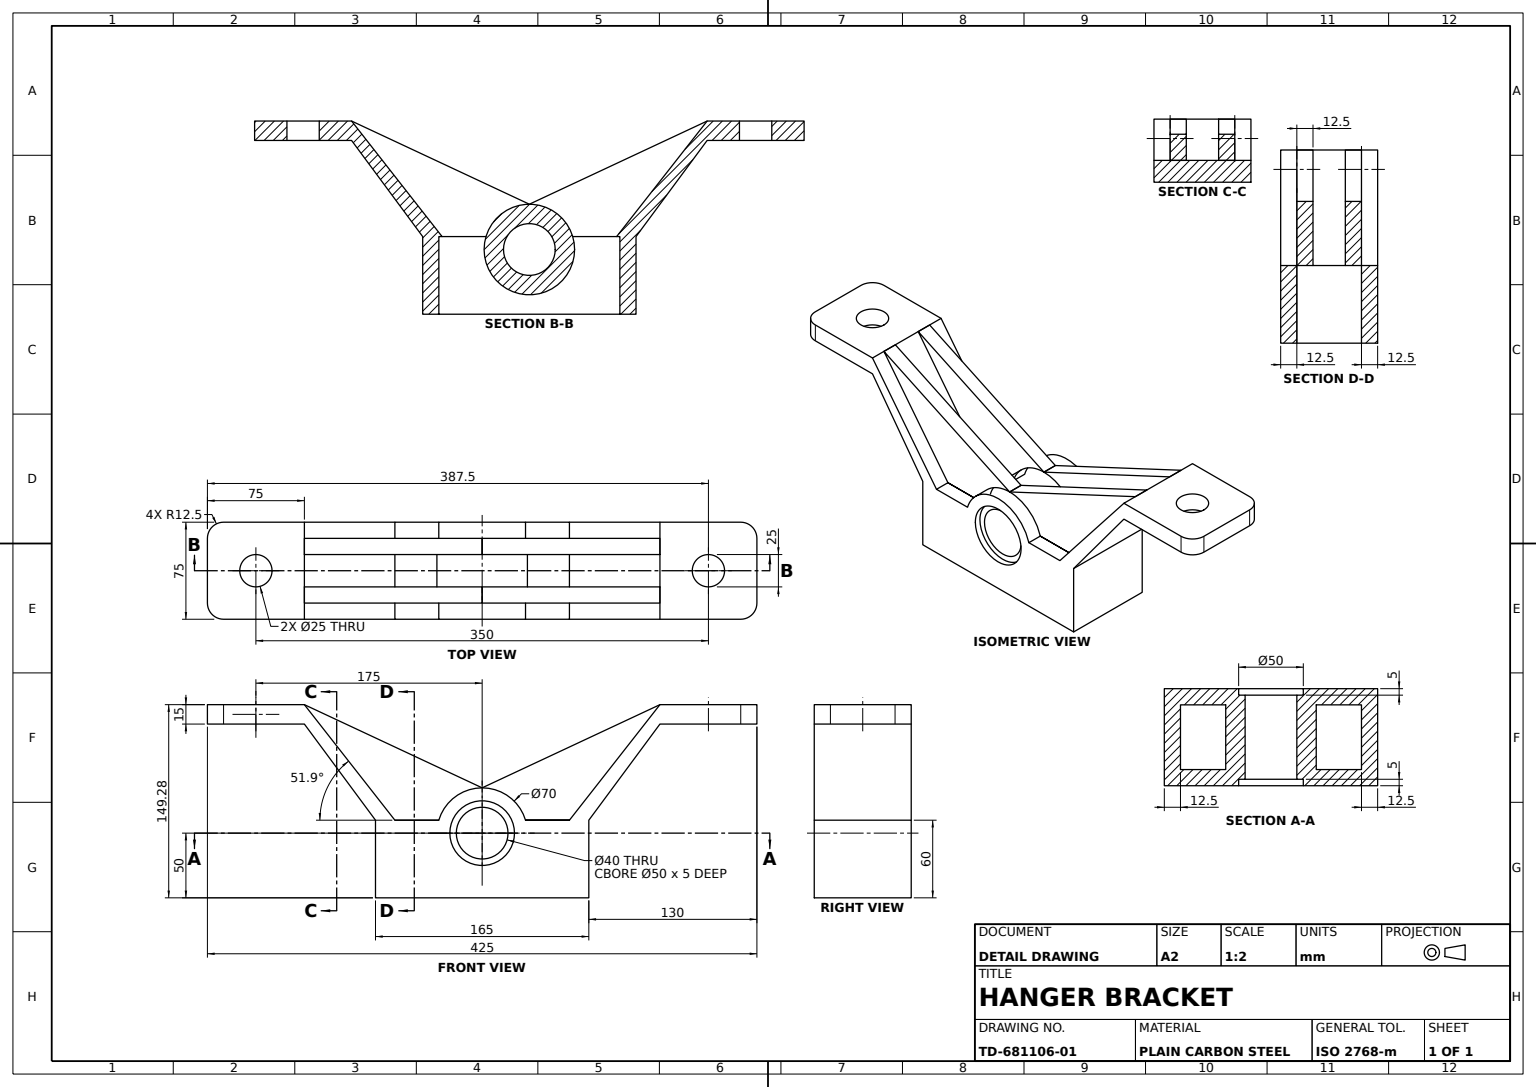
solid
v1 (-137.5,149.280992,12.5)
v2 (-67.5,60,12.5)
e1 v1 v2 LINE
v3 (0,85,12.5)
e2 v3 v1 LINE
v4 (-33.54102,60,12.5)
e3 v4 v3 CIRCLE(AX(P(0,50,12.5),D(0,0,-1),D(-1,0,0)),35)
e4 v2 v4 LINE
face PLANE(AX(P(0,50,12.5),D(0,0,-1),D(-1,0,0))) [-e1 -e2 -e3 -e4]
v5 (-137.5,149.280992,25)
v6 (-67.5,60,25)
e5 v5 v6 LINE
e6 v1 v5 LINE
e7 v2 v6 LINE
face PLANE(AX(P(-137.5,149.280992,12.5),D(-0.786957449,-0.617007272,0),D(0.617007272,-0.786957449,0))) [-e5 -e6 e1 e7]
v7 (0,85,25)
e8 v3 v7 LINE
v8 (-33.54102,60,25)
e9 v8 v7 CIRCLE(AX(P(0,50,25),D(0,0,-1),D(-1,0,0)),35)
e10 v4 v8 LINE
face CYL(AX(P(0,50,12.5),D(0,0,1),D(1,0,0)),35) rev [e3 e8 -e9 -e10]
e11 v7 v5 LINE
e12 v6 v8 LINE
face PLANE(AX(P(0,50,25),D(0,0,-1),D(-1,0,0))) rev [e11 e5 e12 e9]
face PLANE(AX(P(-137.5,149.280992,12.5),D(0.423503881,0.905894289,0),D(-0.905894289,0.423503881,0))) [-e8 e2 e6 -e11]
face PLANE(AX(P(-67.5,60,12.5),D(0,-1,0),D(0,0,-1))) [e4 e10 -e12 -e7]
solid
v9 (137.5,149.280992,-12.5)
v10 (137.5,149.280992,-25)
e13 v9 v10 LINE
v11 (67.5,60,-12.5)
e14 v9 v11 LINE
v12 (67.5,60,-25)
e15 v11 v12 LINE
e16 v10 v12 LINE
face PLANE(AX(P(137.5,149.280992,-12.5),D(0.786957449,-0.617007272,0),D(-0.617007272,-0.786957449,0))) [-e13 e14 e15 -e16]
v13 (0,85,-12.5)
e17 v13 v9 LINE
v14 (33.54102,60,-12.5)
e18 v14 v13 CIRCLE(AX(P(0,50,-12.5),D(0,0,1),D(1,0,0)),35)
e19 v11 v14 LINE
face PLANE(AX(P(0,50,-12.5),D(0,0,1),D(1,0,0))) [-e14 -e17 -e18 -e19]
v15 (0,85,-25)
e20 v15 v10 LINE
e21 v13 v15 LINE
face PLANE(AX(P(137.5,149.280992,-12.5),D(-0.423503881,0.905894289,0),D(0.905894289,0.423503881,0))) [e17 e13 -e20 -e21]
v16 (33.54102,60,-25)
e22 v16 v15 CIRCLE(AX(P(0,50,-25),D(0,0,1),D(1,0,0)),35)
e23 v14 v16 LINE
face CYL(AX(P(0,50,-12.5),D(0,0,-1),D(-1,0,0)),35) rev [e21 -e22 -e23 e18]
e24 v12 v16 LINE
face PLANE(AX(P(67.5,60,-12.5),D(0,-1,0),D(0,0,1))) [-e24 -e15 e19 e23]
face PLANE(AX(P(0,50,-25),D(0,0,1),D(1,0,0))) rev [e20 e16 e24 e22]
solid
v17 (-200,149.280992,37.5)
v18 (-200,134.280992,37.5)
e25 v17 v18 LINE
v19 (-212.5,149.280992,25)
e26 v19 v17 CIRCLE(AX(P(-200,149.280992,25),D(0,1,0),D(-1,0,0)),12.5)
v20 (-212.5,134.280992,25)
e27 v20 v19 LINE
e28 v18 v20 CIRCLE(AX(P(-200,134.280992,25),D(0,-1,0),D(0,0,-1)),12.5)
face CYL(AX(P(-200,60,25),D(0,1,0),D(0,0,1)),12.5) [-e25 -e26 -e27 -e28]
v21 (-187.5,134.280992,0)
v22 (-162.5,134.280992,0)
e29 v21 v22 CIRCLE(AX(P(-175,134.280992,0),D(0,-1,0),D(0,0,-1)),12.5)
e30 v22 v21 CIRCLE(AX(P(-175,134.280992,0),D(0,-1,0),D(0,0,-1)),12.5)
v23 (-212.5,134.280992,-25)
e31 v23 v20 LINE
v24 (-200,134.280992,-37.5)
e32 v23 v24 CIRCLE(AX(P(-200,134.280992,-25),D(0,-1,0),D(0,0,-1)),12.5)
v25 (-137.5,134.280992,-37.5)
e33 v24 v25 LINE
v26 (-137.5,134.280992,37.5)
e34 v25 v26 LINE
e35 v18 v26 LINE
face PLANE(AX(P(-212.5,134.280992,-37.5),D(0,-1,0),D(0,0,-1))) [-e29 -e30] [e28 -e31 e32 e33 e34 -e35]
v27 (-67.5,60,37.5)
v28 (-33.54102,60,37.5)
e36 v27 v28 LINE
v29 (-33.54102,60,25)
e37 v29 v28 LINE
v30 (-67.5,60,25)
e38 v30 v29 LINE
e39 v30 v27 LINE
face PLANE(AX(P(0,60,0),D(0,1,0),D(0,0,1))) [e36 -e37 -e38 e39]
v31 (-187.5,149.280992,0)
v32 (-162.5,149.280992,0)
e40 v31 v32 CIRCLE(AX(P(-175,149.280992,0),D(0,1,0),D(-1,0,0)),12.5)
e41 v32 v31 CIRCLE(AX(P(-175,149.280992,0),D(0,1,0),D(-1,0,0)),12.5)
v33 (-212.5,149.280992,-25)
e42 v33 v19 LINE
v34 (-137.5,149.280992,37.5)
e43 v34 v17 LINE
v35 (-137.5,149.280992,-37.5)
e44 v35 v34 LINE
v36 (-200,149.280992,-37.5)
e45 v35 v36 LINE
e46 v36 v33 CIRCLE(AX(P(-200,149.280992,-25),D(0,1,0),D(-1,0,0)),12.5)
face PLANE(AX(P(-137.5,149.280992,-37.5),D(0,1,0),D(-1,0,0))) [-e40 -e41] [e42 e26 -e43 -e44 e45 e46]
v37 (25,50,32.5)
v38 (-25,50,32.5)
e47 v37 v38 CIRCLE(AX(P(0,50,32.5),D(0,0,1),D(1,0,0)),25)
e48 v38 v37 CIRCLE(AX(P(0,50,32.5),D(0,0,1),D(1,0,0)),25)
v39 (-20,50,32.5)
v40 (20,50,32.5)
e49 v39 v40 CIRCLE(AX(P(0,50,32.5),D(0,0,1),D(1,0,0)),20)
e50 v40 v39 CIRCLE(AX(P(0,50,32.5),D(0,0,1),D(1,0,0)),20)
face PLANE(AX(P(0,50,32.5),D(0,0,1),D(1,0,0))) [e47 e48] [-e49 -e50]
v41 (-70,60,-25)
v42 (-70,60,25)
e51 v41 v42 LINE
v43 (-67.5,60,-25)
e52 v43 v41 LINE
e53 v43 v30 LINE
e54 v42 v30 LINE
face PLANE(AX(P(-82.5,60,-37.5),D(0,-1,0),D(0,0,-1))) [-e51 -e52 e53 -e54]
e55 v33 v23 LINE
face PLANE(AX(P(-212.5,149.280992,-37.5),D(-1,0,0),D(0,0,1))) [e31 e27 -e42 e55]
v44 (-20,50,-32.5)
e56 v44 v39 LINE
v45 (20,50,-32.5)
e57 v45 v40 LINE
e58 v44 v45 CIRCLE(AX(P(0,50,-32.5),D(0,0,1),D(-1,0,0)),20)
face CYL(AX(P(0,50,-76.5),D(0,0,1),D(1,0,0)),20) rev [e56 e49 -e57 -e58]
e59 v45 v44 CIRCLE(AX(P(0,50,-32.5),D(0,0,1),D(-1,0,0)),20)
face CYL(AX(P(0,50,-76.5),D(0,0,1),D(1,0,0)),20) rev [-e59 e57 e50 -e56]
v46 (-25,50,37.5)
e60 v38 v46 LINE
v47 (25,50,37.5)
e61 v37 v47 LINE
e62 v47 v46 CIRCLE(AX(P(0,50,37.5),D(0,0,1),D(1,0,0)),25)
face CYL(AX(P(0,50,32.5),D(0,0,1),D(1,0,0)),25) rev [-e60 -e47 e61 e62]
v48 (-70,0,25)
v49 (70,0,25)
e63 v48 v49 LINE
v50 (70,0,-25)
e64 v49 v50 LINE
v51 (-70,0,-25)
e65 v50 v51 LINE
e66 v51 v48 LINE
v52 (82.5,0,37.5)
v53 (82.5,0,-37.5)
e67 v52 v53 LINE
v54 (-82.5,0,37.5)
e68 v54 v52 LINE
v55 (-82.5,0,-37.5)
e69 v55 v54 LINE
e70 v53 v55 LINE
face PLANE(AX(P(0,0,0),D(0,1,0),D(0,0,1))) rev [e63 e64 e65 e66] [-e67 -e68 -e69 -e70]
v56 (-25,50,-32.5)
v57 (25,50,-32.5)
e71 v56 v57 CIRCLE(AX(P(0,50,-32.5),D(0,0,-1),D(-1,0,0)),25)
e72 v57 v56 CIRCLE(AX(P(0,50,-32.5),D(0,0,-1),D(-1,0,0)),25)
face PLANE(AX(P(0,50,-32.5),D(0,0,-1),D(-1,0,0))) [e58 e59] [e71 e72]
v58 (162.5,149.280992,0)
v59 (187.5,149.280992,0)
e73 v58 v59 CIRCLE(AX(P(175,149.280992,0),D(0,1,0),D(-1,0,0)),12.5)
e74 v59 v58 CIRCLE(AX(P(175,149.280992,0),D(0,1,0),D(-1,0,0)),12.5)
v60 (200,149.280992,37.5)
v61 (212.5,149.280992,25)
e75 v60 v61 CIRCLE(AX(P(200,149.280992,25),D(0,1,0),D(-1,0,0)),12.5)
v62 (212.5,149.280992,-25)
e76 v62 v61 LINE
v63 (200,149.280992,-37.5)
e77 v62 v63 CIRCLE(AX(P(200,149.280992,-25),D(0,1,0),D(-1,0,0)),12.5)
v64 (137.5,149.280992,-37.5)
e78 v63 v64 LINE
v65 (137.5,149.280992,37.5)
e79 v64 v65 LINE
e80 v60 v65 LINE
face PLANE(AX(P(137.5,149.280992,-37.5),D(0,1,0),D(-1,0,0))) [-e73 -e74] [e75 -e76 e77 e78 e79 -e80]
e81 v22 v32 LINE
e82 v21 v31 LINE
face CYL(AX(P(-175,74.280992,0),D(0,1,0),D(-1,0,0)),12.5) rev [-e81 e30 e82 e40]
e83 v41 v51 LINE
e84 v42 v48 LINE
face PLANE(AX(P(-70,60,-37.5),D(1,0,0),D(0,0,-1))) [-e66 -e83 e51 e84]
v66 (200,134.280992,37.5)
e85 v66 v60 LINE
v67 (212.5,134.280992,25)
e86 v67 v66 CIRCLE(AX(P(200,134.280992,25),D(0,-1,0),D(0,0,-1)),12.5)
e87 v61 v67 LINE
face CYL(AX(P(200,60,25),D(0,-1,0),D(0,0,-1)),12.5) [-e75 -e85 -e86 -e87]
v68 (25,50,-37.5)
v69 (-25,50,-37.5)
e88 v68 v69 CIRCLE(AX(P(0,50,-37.5),D(0,0,-1),D(-1,0,0)),25)
e89 v69 v68 CIRCLE(AX(P(0,50,-37.5),D(0,0,-1),D(-1,0,0)),25)
v70 (200,134.280992,-37.5)
e90 v63 v70 LINE
v71 (137.5,134.280992,-37.5)
e91 v71 v70 LINE
v72 (82.5,60,-37.5)
e92 v72 v71 LINE
e93 v72 v53 LINE
v73 (-82.5,60,-37.5)
e94 v73 v55 LINE
e95 v25 v73 LINE
e96 v24 v36 LINE
v74 (-67.5,60,-37.5)
e97 v74 v35 LINE
v75 (-33.54102,60,-37.5)
e98 v75 v74 LINE
v76 (33.54102,60,-37.5)
e99 v76 v75 CIRCLE(AX(P(0,50,-37.5),D(0,0,1),D(1,0,0)),35)
v77 (67.5,60,-37.5)
e100 v77 v76 LINE
e101 v64 v77 LINE
face PLANE(AX(P(82.5,60,-37.5),D(0,0,1),D(1,0,0))) rev [-e88 -e89] [-e78 e90 -e91 -e92 e93 e70 -e94 -e95 -e33 e96 -e45 -e97 -e98 -e99 -e100 -e101]
e102 v56 v69 LINE
e103 v57 v68 LINE
face CYL(AX(P(0,50,-32.5),D(0,0,-1),D(-1,0,0)),25) rev [e88 -e102 -e72 e103]
v78 (33.54102,60,25)
v79 (67.5,60,25)
e104 v78 v79 LINE
v80 (70,60,25)
e105 v79 v80 LINE
e106 v80 v49 LINE
v81 (-35,50,25)
e107 v81 v29 CIRCLE(AX(P(0,50,25),D(0,0,-1),D(-1,0,0)),35)
v82 (35,50,25)
e108 v82 v81 CIRCLE(AX(P(0,50,25),D(0,0,-1),D(-1,0,0)),35)
e109 v78 v82 CIRCLE(AX(P(0,50,25),D(0,0,-1),D(-1,0,0)),35)
face PLANE(AX(P(-82.5,60,25),D(0,0,-1),D(-1,0,0))) [e104 e105 e106 -e63 -e84 e54 e38 -e107 -e108 -e109]
v83 (35,50,-25)
v84 (33.54102,60,-25)
e110 v83 v84 CIRCLE(AX(P(0,50,-25),D(0,0,1),D(1,0,0)),35)
e111 v84 v76 LINE
v85 (-33.54102,60,-25)
e112 v75 v85 LINE
v86 (-35,50,-25)
e113 v85 v86 CIRCLE(AX(P(0,50,-25),D(0,0,1),D(1,0,0)),35)
e114 v86 v81 LINE
v87 (33.54102,60,37.5)
e115 v87 v28 CIRCLE(AX(P(0,50,37.5),D(0,0,1),D(1,0,0)),35)
e116 v87 v78 LINE
e117 v83 v82 LINE
face CYL(AX(P(0,50,-37.5),D(0,0,1),D(1,0,0)),35) [e110 e111 e99 e112 e113 e114 e107 e37 -e115 e116 e109 -e117]
e118 v46 v47 CIRCLE(AX(P(0,50,37.5),D(0,0,1),D(1,0,0)),25)
v88 (-82.5,60,37.5)
e119 v26 v88 LINE
e120 v88 v54 LINE
v89 (82.5,60,37.5)
e121 v89 v52 LINE
v90 (137.5,134.280992,37.5)
e122 v89 v90 LINE
e123 v90 v66 LINE
v91 (67.5,60,37.5)
e124 v65 v91 LINE
e125 v87 v91 LINE
e126 v27 v34 LINE
face PLANE(AX(P(-82.5,60,37.5),D(0,0,-1),D(-1,0,0))) rev [-e118 -e62] [e119 e120 e68 -e121 e122 e123 e85 e80 e124 -e125 e115 -e36 e126 e43 e25 e35]
e127 v74 v43 LINE
e128 v85 v43 LINE
face PLANE(AX(P(0,60,0),D(0,1,0),D(0,0,1))) [-e112 e98 e127 -e128]
e129 v86 v83 CIRCLE(AX(P(0,50,-25),D(0,0,1),D(1,0,0)),35)
face CYL(AX(P(0,50,-37.5),D(0,0,1),D(1,0,0)),35) [e108 -e114 e129 e117]
face CYL(AX(P(0,50,-32.5),D(0,0,-1),D(-1,0,0)),25) rev [-e71 e102 e89 -e103]
e130 v79 v91 LINE
v92 (67.5,60,-25)
e131 v77 v92 LINE
e132 v92 v79 LINE
face PLANE(AX(P(137.5,149.280992,-37.5),D(-0.786957449,0.617007272,0),D(-0.617007272,-0.786957449,0))) [e130 -e124 -e79 e101 e131 e132]
v93 (187.5,134.280992,0)
v94 (162.5,134.280992,0)
e133 v93 v94 CIRCLE(AX(P(175,134.280992,0),D(0,-1,0),D(0,0,-1)),12.5)
e134 v94 v93 CIRCLE(AX(P(175,134.280992,0),D(0,-1,0),D(0,0,-1)),12.5)
e135 v71 v90 LINE
v95 (212.5,134.280992,-25)
e136 v70 v95 CIRCLE(AX(P(200,134.280992,-25),D(0,-1,0),D(0,0,-1)),12.5)
e137 v95 v67 LINE
face PLANE(AX(P(212.5,134.280992,-37.5),D(0,-1,0),D(0,0,-1))) [-e133 -e134] [-e123 -e135 e91 e136 e137 e86]
e138 v73 v88 LINE
face PLANE(AX(P(-82.5,60,-37.5),D(1,0,0),D(0,0,-1))) rev [-e138 e94 e69 -e120]
face CYL(AX(P(-175,74.280992,0),D(0,1,0),D(-1,0,0)),12.5) rev [e81 e41 -e82 e29]
v96 (70,60,-25)
e139 v80 v96 LINE
e140 v96 v92 LINE
face PLANE(AX(P(82.5,60,-37.5),D(0,-1,0),D(0,0,-1))) [-e139 -e105 -e132 -e140]
face CYL(AX(P(-200,149.280992,-25),D(0,1,0),D(0,0,1)),12.5) [-e55 -e46 -e96 -e32]
e141 v89 v72 LINE
face PLANE(AX(P(137.5,134.280992,-37.5),D(0.803675979,-0.595067157,0),D(0.595067157,0.803675979,0))) [e135 -e122 e141 e92]
face PLANE(AX(P(-137.5,134.280992,-37.5),D(-0.803675979,-0.595067157,0),D(0.595067157,-0.803675979,0))) [e95 e138 -e119 -e34]
e142 v94 v58 LINE
e143 v93 v59 LINE
face CYL(AX(P(175,74.280992,0),D(0,1,0),D(-1,0,0)),12.5) rev [e133 e142 e73 -e143]
e144 v92 v84 LINE
face PLANE(AX(P(0,60,0),D(0,1,0),D(0,0,1))) [-e111 -e144 -e131 e100]
face PLANE(AX(P(-137.5,149.280992,-37.5),D(0.786957449,0.617007272,0),D(-0.617007272,0.786957449,0))) [-e127 e97 e44 -e126 -e39 -e53]
e145 v95 v62 LINE
face PLANE(AX(P(212.5,149.280992,-37.5),D(1,0,0),D(0,0,-1))) [e87 -e137 e145 e76]
face PLANE(AX(P(82.5,60,0),D(-1,0,0),D(0,0,1))) rev [e121 e67 -e93 -e141]
e146 v96 v50 LINE
face PLANE(AX(P(82.5,60,-25),D(0,0,1),D(1,0,0))) [-e129 -e113 e128 e52 e83 -e65 -e146 e140 e144 -e110]
face PLANE(AX(P(0,60,0),D(0,1,0),D(0,0,1))) [-e130 -e104 -e116 e125]
face CYL(AX(P(200,149.280992,-25),D(0,-1,0),D(0,0,-1)),12.5) [-e90 -e77 -e145 -e136]
face PLANE(AX(P(70,60,0),D(-1,0,0),D(0,0,1))) [e139 e146 -e64 -e106]
face CYL(AX(P(0,50,32.5),D(0,0,1),D(1,0,0)),25) rev [-e61 -e48 e60 e118]
face CYL(AX(P(175,74.280992,0),D(0,1,0),D(-1,0,0)),12.5) rev [-e142 e134 e143 e74]
solid
v97 (-33.54102,60,-12.5)
v98 (0,85,-12.5)
e147 v97 v98 CIRCLE(AX(P(0,50,-12.5),D(0,0,-1),D(-1,0,0)),35)
v99 (-137.5,149.280992,-12.5)
e148 v98 v99 LINE
v100 (-67.5,60,-12.5)
e149 v99 v100 LINE
e150 v100 v97 LINE
face PLANE(AX(P(0,50,-12.5),D(0,0,1),D(-1,0,0))) [e147 e148 e149 e150]
v101 (-33.54102,60,-25)
e151 v97 v101 LINE
v102 (-67.5,60,-25)
e152 v100 v102 LINE
e153 v102 v101 LINE
face PLANE(AX(P(-67.5,60,-12.5),D(0,-1,0),D(0,0,1))) [-e151 -e150 e152 e153]
v103 (0,85,-25)
v104 (-137.5,149.280992,-25)
e154 v103 v104 LINE
e155 v99 v104 LINE
e156 v98 v103 LINE
face PLANE(AX(P(-137.5,149.280992,-12.5),D(0.423503881,0.905894289,0),D(-0.905894289,0.423503881,0))) [e154 -e155 -e148 e156]
e157 v104 v102 LINE
face PLANE(AX(P(-137.5,149.280992,-12.5),D(-0.786957449,-0.617007272,0),D(0.617007272,-0.786957449,0))) [-e152 -e149 e155 e157]
e158 v101 v103 CIRCLE(AX(P(0,50,-25),D(0,0,-1),D(-1,0,0)),35)
face PLANE(AX(P(0,50,-25),D(0,0,1),D(-1,0,0))) rev [-e154 -e158 -e153 -e157]
face CYL(AX(P(0,50,-12.5),D(0,0,-1),D(1,0,0)),35) rev [e158 -e156 -e147 e151]
solid
v105 (33.54102,60,25)
v106 (0,85,25)
e159 v105 v106 CIRCLE(AX(P(0,50,25),D(0,0,1),D(1,0,0)),35)
v107 (0,85,12.5)
e160 v107 v106 LINE
v108 (33.54102,60,12.5)
e161 v108 v107 CIRCLE(AX(P(0,50,12.5),D(0,0,1),D(1,0,0)),35)
e162 v108 v105 LINE
face CYL(AX(P(0,50,12.5),D(0,0,1),D(-1,0,0)),35) rev [e159 -e160 -e161 e162]
v109 (137.5,149.280992,12.5)
v110 (67.5,60,12.5)
e163 v109 v110 LINE
e164 v110 v108 LINE
e165 v107 v109 LINE
face PLANE(AX(P(0,50,12.5),D(0,0,-1),D(1,0,0))) [e163 e164 e161 e165]
v111 (67.5,60,25)
e166 v111 v105 LINE
v112 (137.5,149.280992,25)
e167 v112 v111 LINE
e168 v106 v112 LINE
face PLANE(AX(P(0,50,25),D(0,0,-1),D(1,0,0))) rev [-e166 -e167 -e168 -e159]
e169 v109 v112 LINE
face PLANE(AX(P(137.5,149.280992,12.5),D(-0.423503881,0.905894289,0),D(0.905894289,0.423503881,0))) [e160 e168 -e169 -e165]
e170 v110 v111 LINE
face PLANE(AX(P(137.5,149.280992,12.5),D(0.786957449,-0.617007272,0),D(-0.617007272,-0.786957449,0))) [-e163 e169 e167 -e170]
face PLANE(AX(P(67.5,60,12.5),D(0,-1,0),D(0,0,-1))) [e170 e166 -e162 -e164]
